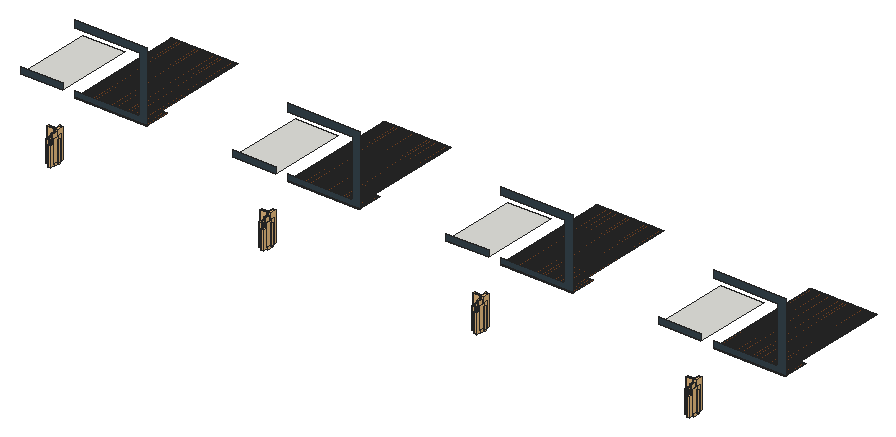
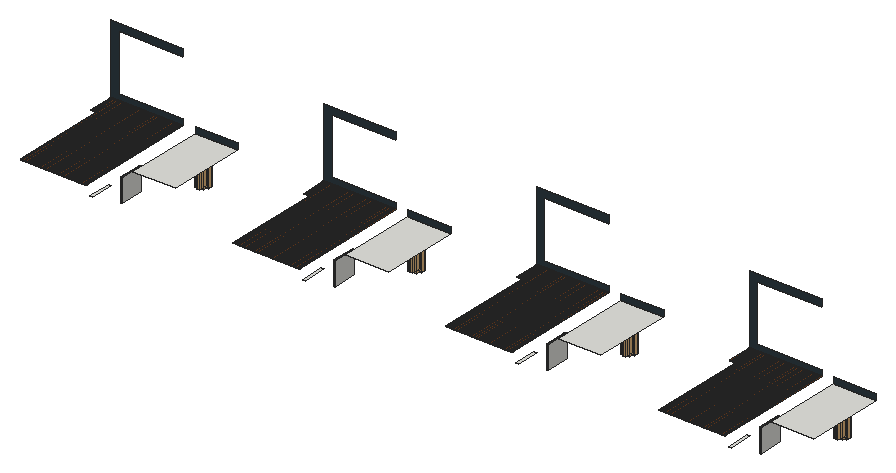
# SketchUp Ruby script. Lengths in inches.
U = 1.inch
M = Sketchup.active_model
def pt(a) = Geom::Point3d.new(a.map { |v| v * U })
def face(e, loops, mat)
  f = e.add_face(loops[0].map { |a| pt(a) })
  loops[1..].each { |l| e.add_face(l.map { |a| pt(a) }).erase! }
  f.material = f.back_material = mat if mat
  f
end
# faces: each face lists its corners as indices into pts; further lists are holes
def faces(e, pts, list, mat = nil) = list.each { |f| face(e, (f[0].is_a?(Array) ? f : [f]).map { |l| l.map { |i| pts[i] } }, mat) }
# xy, xz, yz: faces in a plane at the given z, y or x. An outline is a flat list of corners, or four numbers for a rectangle; further outlines are holes
def ring(l) = l.size == 4 ? [[l[0], l[1]], [l[2], l[1]], [l[2], l[3]], [l[0], l[3]]] : l.each_slice(2).to_a
def flat(e, list, mat, &to3) = list.each { |f| face(e, (f[0].is_a?(Array) ? f : [f]).map { |l| ring(l).map { |u, v| to3.(u, v) } }, mat) }
def xy(e, z, list, mat = nil) = flat(e, list, mat) { |x, y| [x, y, z] }
def xz(e, y, list, mat = nil) = flat(e, list, mat) { |x, z| [x, y, z] }
def yz(e, x, list, mat = nil) = flat(e, list, mat) { |y, z| [x, y, z] }
def lines(e, pts, list) = list.each { |a, b| e.add_line(pt(pts[a]), pt(pts[b])) }
# prism: a flat outline (further loops are holes) pulled along v
def prism(e, loops, v, mat = nil)
  f = face(e, loops, mat); d = Geom::Vector3d.new(v.map { |x| x * U })
  f.pushpull(f.normal.samedirection?(d) ? d.length : -d.length)
end
def box(e, o, s, mat = nil) = prism(e, [[o, [o[0] + s[0], o[1], o[2]], [o[0] + s[0], o[1] + s[1], o[2]], [o[0], o[1] + s[1], o[2]]]], [0, 0, s[2]], mat)
def at(x, y, z, deg = 0) = Geom::Transformation.translation(pt([x, y, z])) * Geom::Transformation.rotation(ORIGIN, Z_AXIS, deg.degrees)
def axes(o, x, y, z) = Geom::Transformation.new([*x, 0, *y, 0, *z, 0, *pt(o).to_a, 1])
def part(name) = M.definitions.add(name)
# library, detail: a bought-in or finely detailed component or shape, given as its bounding box
def library(name, o, s) = part(name).tap { |d| box(d.entities, o, s) }
def detail(e, o, s) = box(e.add_group.entities, o, s)
def put(e, d, t, mat = nil) = e.add_instance(d, t).tap { |i| i.material = mat if mat }
def group(e, t, mat = nil) = e.add_group.tap { |g| g.transformation = t; g.material = mat if mat }.entities
root = M.entities
M.materials.add("1480 AP K099 Starless Night-N").color = [54, 68, 77]
M.materials.add("Glass_Tinted_Gray").color = [0, 0, 0]
M.materials["Glass_Tinted_Gray"].alpha = 0.125
M.materials.add("POT_TEXTURE_1").color = [172, 172, 172]
M.materials.add("[0135_DarkGray]1").color = [81, 81, 81]
M.materials.add("[Mirror 02]").color = [229, 229, 229]
M.materials.add("[Terrazzo Light Blue]").color = [196, 214, 227]
M.materials.add("[Wood Cherry Original]").color = [152, 86, 42]
M.materials.add("white_concrete_pot1").color = [212, 211, 204]
c1 = library("Group\#12",[-312.76,2118.02,370.79],[80.37,61.43,57.53])
c2 = library("Group\#37",[-146.29,2044.53,349.125],[81,53.32,37.9])
c3 = library("Group\#85",[-236.03,2064.57,238.29],[378.97,266.89,1422.96])
c4 = library("Group\#21",[-392.38,2142.99,345.23],[79.77,60.6,39.05])
c5 = library("Group\#52",[-390.04,2074.71,363.78],[77.3,84.83,61.55])
c6 = library("Group\#25",[-389.63,2051.04,359.41],[56.81,81.38,37.86])
c7 = library("Group\#29",[-362.86,1963.26,351.01],[55.56,80.44,37.9])
c8 = library("Group\#36",[-200.52,1998.86,370.22],[77.15,68.38,35.39])
c9 = library("Group\#48",[-480.58,1843.32,11.96],[467.85,466.24,378.92])
c10 = library("Group\#22",[-433.57,2042.61,369.7],[71.79,72.8,37.85])
c11 = library("Group\#19",[-148.5,2084.1,354.63],[73.89,71.73,39.48])
c12 = library("Group\#63",[-372.4375,2154.5,374],[76.125,67.08,39.0625])
c13 = library("Group\#64",[-275.5,2156.34,352.11],[71.39,73.27,44.69])
c14 = library("Group\#42",[-143.56,2061.14,371.42],[79.79,63.19,51.3])
c15 = library("Group\#51",[-363.89,1895.22,354.63],[76.92,66.54,39.48])
c16 = library("Group\#44",[-145.08,2015.32,369.99],[82.29,54.05,37.9])
c17 = library("Group\#60",[-315.77,2202.04,371],[80.74,54.44,37.85])
c18 = library("Group\#53",[-419.21,1941.11,355.02],[73.1,71.21,39.06])
c19 = library("Group\#56",[-229.79,1894.04,351.01],[79.82,63.55,37.9])
c20 = library("Group\#70",[-234.26,2180.97,367.05],[50.63,74.65,43.95])
c21 = library("Group\#72",[-904.81,1865.01,156.3],[624.43,217.34,1227.7])
c22 = library("Group\#73",[-312.51,1611.52,263.78],[120.52,408.52,1275.1])
c23 = library("Group\#75",[-571.16,1736.08,232.33],[294.08,306.57,1438.75])
c24 = library("Group\#77",[-273.21,1593.22,47.51],[374.54,419.07,1416.6])
c25 = library("Group\#16",[-202.35,1900.5,372.29],[58.53,80.11,50.06])
c26 = library("Group\#24",[-432.01,1984.38,372.6875],[64.1,75.95,39.0625])
c27 = library("Group\#41",[-310.7,1952.62,354.63],[79.53,58.52,39.48])
c28 = library("Group\#23",[-374.28,1979.7,369.99],[51.81,82.66,37.9])
c29 = library("Group\#58",[-397.18,1916.74,372.44],[70.02,74.57,49.25])
c30 = library("Group\#66",[-236.3,2186.8,344.47],[79.26,62.91,39.06])
c31 = library("Group\#15",[-161.07,2117.49,373.61],[81.25,53.73,39.48])
c32 = library("Group\#71",[-431.9,1883.46,368.72],[373.65,376.39,18.61])
c33 = library("Group\#40",[-340.96,1970.4,361.28],[81.22,51.59,61.62])
c34 = library("Group\#46",[-272.7,1884.51,369.99],[80.39,55.87,37.9])
c35 = library("Group\#35",[-330.83,2117.69,370.2],[61.83,80.2,35.55])
c36 = library("Group\#69",[-366.3125,2177.8,359.41],[79.9,61.23,37.86])
c37 = library("Group\#28",[-435.875,2067.96,347.82],[58.32,80.53,38.29])
c38 = library("Group\#65",[-183.79,2161.45,371.25],[72.43,70.21,54.35])
c39 = library("Group\#76",[-208.23,2037.18,75.37],[621.09,225.61,1251.82])
c40 = library("Group\#79",[-675.58,1862.05,152.55],[378.81,196.01,1743.84])
c41 = library("Group\#80",[-257.06,2048.08,160.05],[394.6,177.93,1743.83])
c42 = library("Group\#82",[-344.84,1500.61,160.55],[176.35,551.19,1921.45])
c43 = library("Group\#83",[-231.77,1913.24,119.96],[448.93,143.84,1582.05])
c44 = library("Group\#84",[-616.67,2098.6,178.29],[331.19,111.16,1177.92])
c45 = library("Group\#78",[-527.15,2088.47,150.96],[267.01,328.12,1599.25])
c46 = library("Group\#87",[-792.12,2067.32,152.13],[549.56,259.52,1931.8])
c47 = library("Group\#88",[-281.17,2118.67,243.77],[133.23,408.71,1313.3])
c48 = part("Potted foliage plant")
g1 = group(c48.entities,at(904.81,-1500.61,-11.96),"white_concrete_pot1")
detail(g1,[-222.14,2117.95,372.07],[61.87,75.41,50.35])
put(c48.entities,c1,at(904.81,-1500.61,-11.96),"white_concrete_pot1")
g2 = group(c48.entities,at(904.81,-1500.61,-11.96),"white_concrete_pot1")
detail(g2,[-313.93,1881.02,351.21],[70.15,73.18,37.2])
g3 = group(c48.entities,at(904.81,-1500.61,-11.96),"white_concrete_pot1")
detail(g3,[-209.1,1970.26,378.89],[50.57,81.04,37.2])
put(c48.entities,c2,at(904.81,-1500.61,-11.96),"white_concrete_pot1")
put(c48.entities,c3,at(904.81,-1500.61,-11.96))
put(c48.entities,c4,at(904.81,-1500.61,-11.96),"white_concrete_pot1")
put(c48.entities,c5,at(904.81,-1500.61,-11.96),"white_concrete_pot1")
put(c48.entities,c6,at(904.81,-1500.61,-11.96),"white_concrete_pot1")
put(c48.entities,c7,at(904.81,-1500.61,-11.96),"white_concrete_pot1")
g4 = group(c48.entities,at(904.81,-1500.61,-11.96),"white_concrete_pot1")
detail(g4,[-129.49,1972.75,359.91],[55.59,80.76,37.2])
put(c48.entities,c8,at(904.81,-1500.61,-11.96),"white_concrete_pot1")
g5 = group(c48.entities,at(904.81,-1500.61,-11.96),"white_concrete_pot1")
detail(g5,[-333.13,1892.25,370.19],[61.39,79.4,37.2])
put(c48.entities,c9,at(904.81,-1500.61,-11.96),"POT_TEXTURE_1")
put(c48.entities,c10,at(904.81,-1500.61,-11.96),"white_concrete_pot1")
put(c48.entities,c11,at(904.81,-1500.61,-11.96),"white_concrete_pot1")
g6 = group(c48.entities,at(904.81,-1500.61,-11.96),"white_concrete_pot1")
detail(g6,[-270.91,2176.57,345.18],[52.11,82.01,38.29])
g7 = group(c48.entities,at(904.81,-1500.61,-11.96),"white_concrete_pot1")
detail(g7,[-195.71,2019.1875,371.11],[58.98,81.18,37.2])
g8 = group(c48.entities,at(904.81,-1500.61,-11.96),"white_concrete_pot1")
detail(g8,[-319.36,2078.81,339.18],[76.07,69.08,39.48])
put(c48.entities,c12,at(904.81,-1500.61,-11.96),"white_concrete_pot1")
put(c48.entities,c13,at(904.81,-1500.61,-11.96),"white_concrete_pot1")
g9 = group(c48.entities,at(904.81,-1500.61,-11.96),"white_concrete_pot1")
detail(g9,[-417.64,2112.53,369.82],[65.44,79.59,38.29])
put(c48.entities,c14,at(904.81,-1500.61,-11.96),"white_concrete_pot1")
put(c48.entities,c15,at(904.81,-1500.61,-11.96),"white_concrete_pot1")
put(c48.entities,c16,at(904.81,-1500.61,-11.96),"white_concrete_pot1")
g10 = group(c48.entities,at(904.81,-1500.61,-11.96),"white_concrete_pot1")
detail(g10,[-240.6,2054.85,378.89],[71.5,72.03,37.2])
put(c48.entities,c17,at(904.81,-1500.61,-11.96),"white_concrete_pot1")
put(c48.entities,c18,at(904.81,-1500.61,-11.96),"white_concrete_pot1")
put(c48.entities,c19,at(904.81,-1500.61,-11.96),"white_concrete_pot1")
g11 = group(c48.entities,at(904.81,-1500.61,-11.96),"white_concrete_pot1")
detail(g11,[-249.82,2117.53,359.91],[58.07,81.25,37.2])
put(c48.entities,c20,at(904.81,-1500.61,-11.96),"white_concrete_pot1")
put(c48.entities,c21,at(904.81,-1500.61,-11.96))
put(c48.entities,c22,at(904.81,-1500.61,-11.96))
put(c48.entities,c23,at(904.81,-1500.61,-11.96))
put(c48.entities,c24,at(904.81,-1500.61,-11.96))
g12 = group(c48.entities,at(904.81,-1500.61,-11.96),"white_concrete_pot1")
detail(g12,[-435.4375,2027.54,350.71],[78.74,62.6,37.86])
put(c48.entities,c25,at(904.81,-1500.61,-11.96),"white_concrete_pot1")
g13 = group(c48.entities,at(904.81,-1500.61,-11.96),"white_concrete_pot1")
detail(g13,[-173.8,2126.25,354.63],[80.17,60.53,39.48])
g14 = group(c48.entities,at(904.81,-1500.61,-11.96),"white_concrete_pot1")
detail(g14,[-222.96,2066.75,359.91],[63.77,78.21,37.2])
put(c48.entities,c26,at(904.81,-1500.61,-11.96),"white_concrete_pot1")
g15 = group(c48.entities,at(904.81,-1500.61,-11.96),"white_concrete_pot1")
detail(g15,[-183.125,1913.38,330.04],[66.78,77.69,39.48])
put(c48.entities,c27,at(904.81,-1500.61,-11.96),"white_concrete_pot1")
g16 = group(c48.entities,at(904.81,-1500.61,-11.96),"white_concrete_pot1")
detail(g16,[-152,1936.85,378.89],[64.46,79.76,37.2])
g17 = group(c48.entities,at(904.81,-1500.61,-11.96),"white_concrete_pot1")
detail(g17,[-284.65,1933.22,373.64],[80.83,55.23,37.2])
put(c48.entities,c28,at(904.81,-1500.61,-11.96),"white_concrete_pot1")
g18 = group(c48.entities,at(904.81,-1500.61,-11.96),"white_concrete_pot1")
detail(g18,[-263.49,1923.54,359.91],[75.98,66.75,37.2])
put(c48.entities,c29,at(904.81,-1500.61,-11.96),"white_concrete_pot1")
g19 = group(c48.entities,at(904.81,-1500.61,-11.96),"white_concrete_pot1")
detail(g19,[-167.97,1940.97,354.63],[66.78,77.7,39.48])
put(c48.entities,c30,at(904.81,-1500.61,-11.96),"white_concrete_pot1")
g20 = group(c48.entities,at(904.81,-1500.61,-11.96),"white_concrete_pot1")
detail(g20,[-214.75,1956.59,330.04],[66.78,77.69,39.48])
put(c48.entities,c31,at(904.81,-1500.61,-11.96),"white_concrete_pot1")
put(c48.entities,c32,at(904.81,-1500.61,-11.96),"white_concrete_pot1")
put(c48.entities,c33,at(904.81,-1500.61,-11.96),"white_concrete_pot1")
g21 = group(c48.entities,at(904.81,-1500.61,-11.96),"white_concrete_pot1")
detail(g21,[-282.5625,1934.21,389.56],[81.1,59.19,35.03])
put(c48.entities,c34,at(904.81,-1500.61,-11.96),"white_concrete_pot1")
g22 = group(c48.entities,at(904.81,-1500.61,-11.96),"white_concrete_pot1")
detail(g22,[-394.5,2036.48,359.91],[79.58,64.84,37.2])
put(c48.entities,c35,at(904.81,-1500.61,-11.96),"white_concrete_pot1")
put(c48.entities,c36,at(904.81,-1500.61,-11.96),"white_concrete_pot1")
put(c48.entities,c37,at(904.81,-1500.61,-11.96),"white_concrete_pot1")
put(c48.entities,c38,at(904.81,-1500.61,-11.96),"white_concrete_pot1")
put(c48.entities,c39,at(904.81,-1500.61,-11.96))
put(c48.entities,c40,at(904.81,-1500.61,-11.96))
put(c48.entities,c41,at(904.81,-1500.61,-11.96))
put(c48.entities,c42,at(904.81,-1500.61,-11.96))
put(c48.entities,c43,at(904.81,-1500.61,-11.96))
put(c48.entities,c44,at(904.81,-1500.61,-11.96))
put(c48.entities,c45,at(904.81,-1500.61,-11.96))
put(c48.entities,c46,at(904.81,-1500.61,-11.96))
put(c48.entities,c47,at(904.81,-1500.61,-11.96))
c49 = part("PENTEK_RP Fineline 50S_Sliding_DoorCase_E1")
box(c49.entities,[0,0,0],[1.51,3.66,99.27],"[0135_DarkGray]1")
c50 = part("PENTEK_RP Fineline 50S_SlidingDooe_Case_E2")
box(c50.entities,[0,0,0],[96.25,3.66,1.51],"[0135_DarkGray]1")
c51 = part("pentek_RP Fineline 50S_SlidingDoor_Case")
put(c51.entities,c49,at(97.76,0,0))
put(c51.entities,c50,at(1.51,0,0))
put(c51.entities,c49,at(0,0,0))
put(c51.entities,c50,at(1.51,0,97.76))
c52 = part("PENTEK_RP Fineline 50S_SlidingDoor_GlazingBead_2")
box(c52.entities,[0,0,0],[0.56,0.59,94.39],"[0135_DarkGray]1")
c53 = part("PENTEK_RP Fineline 50S_SlidingDoor_Glass")
box(c53.entities,[0,0,0],[46.58,0.16,94.39],"Glass_Tinted_Gray")
c54 = part("PENTEK_RP Fineline 50S_SlidingDoor_GlazingBead")
box(c54.entities,[0,0,0],[45.47,0.59,0.56],"[0135_DarkGray]1")
c55 = part("PENTEK_RP Fineline 50S_SlidingDoor_Leaf_E1")
xy(c55.entities,0,[[0,0,0.93,1.97],[0.93,1.57,1.49,1.97]],"[0135_DarkGray]1")
xy(c55.entities,96.25,[[0,0,0.93,0,0.93,1.57,1.49,1.57,1.49,1.97,0,1.97]],"[0135_DarkGray]1")
xz(c55.entities,0,[[0,0,0.93,96.25]],"[0135_DarkGray]1")
xz(c55.entities,1.57,[[0.93,0,1.49,95.32],[0.93,95.32,1.49,96.25]],"[0135_DarkGray]1")
xz(c55.entities,1.97,[[0,0,1.49,96.25]],"[0135_DarkGray]1")
yz(c55.entities,0,[[0,0,1.97,96.25]],"[0135_DarkGray]1")
yz(c55.entities,0.93,[[0,0,1.57,0.93],[0,0.93,1.57,95.32],[0,95.32,1.57,96.25]],"[0135_DarkGray]1")
yz(c55.entities,1.49,[[1.57,0,1.97,95.32],[1.57,95.32,1.97,96.25]],"[0135_DarkGray]1")
c56 = part("PENTEK_RP Fineline 50S_SlidingDoor_Leaf_E2")
xy(c56.entities,0,[[0,0,0,1.57,0.56,1.57,0.56,1.97,46.02,1.97,46.02,1.57,46.58,1.57,46.58,0]],"[0135_DarkGray]1")
xy(c56.entities,0.93,[[0,0,46.58,1.57]],"[0135_DarkGray]1")
xy(c56.entities,1.49,[[0.56,1.57,46.02,1.97]],"[0135_DarkGray]1")
xz(c56.entities,0,[[0,0,46.58,0.93]],"[0135_DarkGray]1")
xz(c56.entities,1.57,[[0,0,0.56,0.93],[46.02,0,46.58,0.93],[0.56,0.93,46.02,1.49]],"[0135_DarkGray]1")
xz(c56.entities,1.97,[[0.56,0,46.02,1.49]],"[0135_DarkGray]1")
yz(c56.entities,0,[[0,0,1.57,0.93]],"[0135_DarkGray]1")
yz(c56.entities,0.56,[[1.57,0,1.97,0.93],[1.57,0.93,1.97,1.49]],"[0135_DarkGray]1")
yz(c56.entities,46.02,[[1.57,0,1.97,0.93],[1.57,0.93,1.97,1.49]],"[0135_DarkGray]1")
yz(c56.entities,46.58,[[0,0,1.57,0.93]],"[0135_DarkGray]1")
c57 = part("PENTEK_RP Fineline S_SlidingDoor_Leaf1")
put(c57.entities,c52,at(0.93,0,0.93))
put(c57.entities,c52,at(46.96,0,0.93))
put(c57.entities,c53,at(1.49,1.42,0.93))
put(c57.entities,c54,at(1.49,0,0.93))
put(c57.entities,c53,at(1.49,0.59,0.93),"[Terrazzo Light Blue]")
put(c57.entities,c55,at(0,0,0))
put(c57.entities,c55,axes([48.44,0,0],[-1,0,0],[0,1,0],[0,0,1]))
put(c57.entities,c56,axes([0.93,0,96.25],[1,0,0],[0,1,0],[0,0,-1]))
put(c57.entities,c56,at(0.93,0,0))
put(c57.entities,c54,at(1.49,0,94.77))
c58 = part("PENTEK_RP Fineline 50S_SlidingDoor_Leaf2")
put(c58.entities,c53,at(1.49,1.42,0.93))
put(c58.entities,c54,at(1.49,0,94.77))
put(c58.entities,c52,at(46.96,0,0.93))
put(c58.entities,c53,at(1.49,0.59,0.93),"[Mirror 02]")
put(c58.entities,c52,at(0.93,0,0.93))
put(c58.entities,c55,at(0,0,0))
put(c58.entities,c55,axes([48.44,0,0],[-1,0,0],[0,1,0],[0,0,1]))
put(c58.entities,c54,at(1.49,0,0.93))
put(c58.entities,c56,axes([0.93,0,96.25],[1,0,0],[0,1,0],[0,0,-1]))
put(c58.entities,c56,at(0.93,0,0))
c59 = part("PENTEK - Slimmest Steel Sliding Door / Window\#1")
put(c59.entities,c51,at(0,-1.88,-0.09))
put(c59.entities,c57,at(1.51,-2.27,1.42))
put(c59.entities,c58,at(49.32,-0.3,1.42))
c60 = part("Group50\#1")
box(c60.entities,[-75,-126,0],[1.18,252,0.24])
c61 = part("Group51\#1")
box(c61.entities,[-73.62,-126,0],[1.18,252,0.24])
c62 = part("Group52\#1")
box(c62.entities,[-72.24,-126,0],[1.18,252,0.24])
c63 = part("Group53\#1")
box(c63.entities,[-70.87,-126,0],[1.18,252,0.24])
c64 = part("Group54\#1")
box(c64.entities,[-69.49,-126,0],[1.18,252,0.24])
c65 = part("Group55\#1")
box(c65.entities,[-68.11,-126,0],[1.18,252,0.24])
c66 = part("Group56\#1")
box(c66.entities,[-66.73,-126,0],[1.18,252,0.24])
c67 = part("Group57\#1")
box(c67.entities,[-65.35,-126,0],[1.18,252,0.24])
c68 = part("Group58\#1")
box(c68.entities,[-63.98,-126,0],[1.18,252,0.24])
c69 = part("Group59\#1")
box(c69.entities,[-62.6,-126,0],[1.18,252,0.24])
c70 = part("Group60\#1")
box(c70.entities,[-61.22,-126,0],[1.18,252,0.24])
c71 = part("Group61\#1")
box(c71.entities,[-59.84,-126,0],[1.18,252,0.24])
c72 = part("Group62\#1")
box(c72.entities,[-58.46,-126,0],[1.18,252,0.24])
c73 = part("Group63\#1")
box(c73.entities,[-57.09,-126,0],[1.18,252,0.24])
c74 = part("Group64\#1")
box(c74.entities,[-55.71,-126,0],[1.18,252,0.24])
c75 = part("Group65\#1")
box(c75.entities,[-54.33,-126,0],[1.18,252,0.24])
c76 = part("Group66\#1")
box(c76.entities,[-52.95,-126,0],[1.18,252,0.24])
c77 = part("Group67\#1")
box(c77.entities,[-51.57,-126,0],[1.18,252,0.24])
c78 = part("Group68\#1")
box(c78.entities,[-50.2,-126,0],[1.18,252,0.24])
c79 = part("Group69\#1")
box(c79.entities,[-48.82,-126,0],[1.18,252,0.24])
c80 = part("Group70\#1")
box(c80.entities,[-47.44,-126,0],[1.18,252,0.24])
c81 = part("Group71\#1")
box(c81.entities,[-46.0625,-126,0],[1.18,252,0.24])
c82 = part("Group72\#1")
box(c82.entities,[-44.69,-126,0],[1.19,252,0.24])
c83 = part("Group73\#1")
box(c83.entities,[-43.31,-126,0],[1.19,252,0.24])
c84 = part("Group74\#1")
box(c84.entities,[-41.93,-126,0],[1.18,252,0.24])
c85 = part("Group75\#1")
box(c85.entities,[-40.55,-126,0],[1.18,252,0.24])
c86 = part("Group76\#1")
box(c86.entities,[-39.17,-126,0],[1.18,252,0.24])
c87 = part("Group77\#1")
box(c87.entities,[-37.8,-126,0],[1.19,252,0.24])
c88 = part("Group78\#1")
box(c88.entities,[-36.42,-126,0],[1.18,252,0.24])
c89 = part("Group79\#1")
box(c89.entities,[-35.04,-126,0],[1.18,252,0.24])
c90 = part("Group80\#1")
box(c90.entities,[-33.66,-126,0],[1.18,252,0.24])
c91 = part("Group81\#1")
box(c91.entities,[-32.28,-126,0],[1.18,252,0.24])
c92 = part("Group82\#1")
box(c92.entities,[-30.91,-126,0],[1.19,252,0.24])
c93 = part("Group83\#1")
box(c93.entities,[-29.53,-126,0],[1.18,252,0.24])
c94 = part("Group84\#1")
box(c94.entities,[-28.15,-126,0],[1.18,252,0.24])
c95 = part("Group85\#1")
box(c95.entities,[-26.77,-126,0],[1.18,252,0.24])
c96 = part("Group86\#1")
box(c96.entities,[-25.39,-126,0],[1.18,252,0.24])
c97 = part("Group87\#1")
box(c97.entities,[-24.02,-126,0],[1.19,252,0.24])
c98 = part("Group88\#1")
box(c98.entities,[-22.64,-126,0],[1.18,252,0.24])
c99 = part("Group89\#1")
box(c99.entities,[-21.26,-126,0],[1.18,252,0.24])
c100 = part("Group90\#1")
box(c100.entities,[-19.88,-126,0],[1.18,252,0.24])
c101 = part("Group91\#1")
box(c101.entities,[-18.5,-126,0],[1.18,252,0.24])
c102 = part("Group92\#1")
box(c102.entities,[-17.125,-126,0],[1.19,252,0.24])
c103 = part("Group93\#1")
box(c103.entities,[-15.75,-126,0],[1.18,252,0.24])
c104 = part("Group94\#1")
box(c104.entities,[-14.37,-126,0],[1.18,252,0.24])
c105 = part("Group95\#1")
box(c105.entities,[-12.99,-126,0],[1.18,252,0.24])
c106 = part("Group96\#1")
box(c106.entities,[-11.61,-126,0],[1.18,252,0.24])
c107 = part("Group97\#1")
box(c107.entities,[-10.24,-126,0],[1.18,252,0.24])
c108 = part("Group98\#1")
box(c108.entities,[-8.86,-126,0],[1.18,252,0.24])
c109 = part("Group99\#1")
box(c109.entities,[-7.48,-126,0],[1.18,252,0.24])
c110 = part("Group100\#1")
box(c110.entities,[-6.1,-126,0],[1.18,252,0.24])
c111 = part("Group101\#1")
box(c111.entities,[-4.72,-126,0],[1.18,252,0.24])
c112 = part("Group102\#1")
box(c112.entities,[-3.35,-126,0],[1.18,252,0.24])
c113 = part("Group103\#1")
box(c113.entities,[-1.97,-126,0],[1.18,252,0.24])
c114 = part("Group104\#1")
box(c114.entities,[-0.59,-126,0],[1.18,252,0.24])
c115 = part("Group105\#1")
box(c115.entities,[0.79,-126,0],[1.18,252,0.24])
c116 = part("Group106\#1")
box(c116.entities,[2.17,-126,0],[1.18,252,0.24])
c117 = part("Group107\#1")
box(c117.entities,[3.54,-126,0],[1.18,252,0.24])
c118 = part("Group108\#1")
box(c118.entities,[4.92,-126,0],[1.18,252,0.24])
c119 = part("Group109\#1")
box(c119.entities,[6.3,-126,0],[1.18,252,0.24])
c120 = part("Group110\#1")
box(c120.entities,[7.68,-126,0],[1.18,252,0.24])
c121 = part("Group111\#1")
box(c121.entities,[9.06,-126,0],[1.18,252,0.24])
c122 = part("Group112\#1")
box(c122.entities,[10.43,-126,0],[1.18,252,0.24])
c123 = part("Group113\#1")
box(c123.entities,[11.8125,-126,0],[1.18,252,0.24])
c124 = part("Group114\#1")
box(c124.entities,[13.1875,-126,0],[1.18,252,0.24])
c125 = part("Group115\#1")
box(c125.entities,[14.57,-126,0],[1.18,252,0.24])
c126 = part("Group116\#1")
box(c126.entities,[15.94,-126,0],[1.19,252,0.24])
c127 = part("Group117\#1")
box(c127.entities,[17.32,-126,0],[1.18,252,0.24])
c128 = part("Group118\#1")
box(c128.entities,[18.7,-126,0],[1.18,252,0.24])
c129 = part("Group119\#1")
box(c129.entities,[20.08,-126,0],[1.18,252,0.24])
c130 = part("Group120\#1")
box(c130.entities,[21.46,-126,0],[1.18,252,0.24])
c131 = part("Group121\#1")
box(c131.entities,[22.83,-126,0],[1.19,252,0.24])
c132 = part("Group122\#1")
box(c132.entities,[24.21,-126,0],[1.18,252,0.24])
c133 = part("Group123\#1")
box(c133.entities,[25.59,-126,0],[1.18,252,0.24])
c134 = part("Group124\#1")
box(c134.entities,[26.97,-126,0],[1.18,252,0.24])
c135 = part("Group125\#1")
box(c135.entities,[28.35,-126,0],[1.18,252,0.24])
c136 = part("Group126\#1")
box(c136.entities,[29.72,-126,0],[1.19,252,0.24])
c137 = part("Group127\#1")
box(c137.entities,[31.1,-126,0],[1.18,252,0.24])
c138 = part("Group128\#1")
box(c138.entities,[32.48,-126,0],[1.18,252,0.24])
c139 = part("Group129\#1")
box(c139.entities,[33.86,-126,0],[1.18,252,0.24])
c140 = part("Group130\#1")
box(c140.entities,[35.24,-126,0],[1.18,252,0.24])
c141 = part("Group131\#1")
box(c141.entities,[36.61,-126,0],[1.19,252,0.24])
c142 = part("Group132\#1")
box(c142.entities,[37.99,-126,0],[1.18,252,0.24])
c143 = part("Group133\#1")
box(c143.entities,[39.37,-126,0],[1.18,252,0.24])
c144 = part("Group134\#1")
box(c144.entities,[40.75,-126,0],[1.18,252,0.24])
c145 = part("Group135\#1")
box(c145.entities,[42.125,-126,0],[1.19,252,0.24])
c146 = part("Group136\#1")
box(c146.entities,[43.5,-126,0],[1.19,252,0.24])
c147 = part("Group137\#1")
box(c147.entities,[44.88,-126,0],[1.18,252,0.24])
c148 = part("Group138\#1")
box(c148.entities,[46.26,-126,0],[1.18,252,0.24])
c149 = part("Group139\#1")
box(c149.entities,[47.64,-126,0],[1.18,252,0.24])
c150 = part("Group140\#1")
box(c150.entities,[49.02,-126,0],[1.18,252,0.24])
c151 = part("Group141\#2")
box(c151.entities,[50.39,-126,0],[1.18,252,0.24])
c152 = part("Group142\#1")
box(c152.entities,[51.77,-126,0],[1.18,252,0.24])
c153 = part("Group143\#1")
box(c153.entities,[53.15,-126,0],[1.18,252,0.24])
c154 = part("Group144\#2")
box(c154.entities,[54.53,-126,0],[1.18,252,0.24])
c155 = part("Group145\#1")
box(c155.entities,[55.91,-126,0],[1.18,252,0.24])
c156 = part("Group146\#1")
box(c156.entities,[57.28,-126,0],[1.18,252,0.24])
c157 = part("Group147\#1")
box(c157.entities,[58.66,-126,0],[1.18,252,0.24])
c158 = part("Group148\#1")
box(c158.entities,[60.04,-126,0],[1.18,252,0.24])
c159 = part("Group149\#1")
box(c159.entities,[61.42,-126,0],[1.18,252,0.24])
c160 = part("Group150\#1")
xy(c160.entities,0,[[62.8,-126,62.8,126,63,126,63,-73.9375,63.98,-73.9375,63.98,-126]])
xy(c160.entities,0.24,[[62.8,-126,63.98,-126,63.98,-73.9375,63,-73.9375,63,126,62.8,126]])
xz(c160.entities,-126,[[62.8,0,63.98,0.24]])
yz(c160.entities,62.8,[[-126,0,126,0.24]])
yz(c160.entities,63.98,[[-126,0,-73.9375,0.24]])
c161 = part("Group151\#1")
box(c161.entities,[64.17,-126,0],[1.18,52.0625,0.24])
c162 = part("Group152\#1")
box(c162.entities,[65.55,-126,0],[1.18,52.0625,0.24])
c163 = part("Group153\#1")
box(c163.entities,[66.93,-126,0],[1.18,52.0625,0.24])
c164 = part("Group154\#1")
box(c164.entities,[68.31,-126,0],[1.18,52.0625,0.24])
c165 = part("Group155\#1")
box(c165.entities,[69.69,-126,0],[1.18,52.0625,0.24])
c166 = part("Group156\#1")
box(c166.entities,[71.0625,-126,0],[1.18,52.0625,0.24])
c167 = part("Group157\#1")
box(c167.entities,[72.44,-126,0],[1.18,52.0625,0.24])
c168 = part("Group158\#1")
box(c168.entities,[73.82,-126,0],[1.18,52.0625,0.24])
c169 = part("Group48\#1")
put(c169.entities,c60,at(0,0,0))
put(c169.entities,c61,at(0,0,0))
put(c169.entities,c62,at(0,0,0))
put(c169.entities,c63,at(0,0,0))
put(c169.entities,c64,at(0,0,0))
put(c169.entities,c65,at(0,0,0))
put(c169.entities,c66,at(0,0,0))
put(c169.entities,c67,at(0,0,0))
put(c169.entities,c68,at(0,0,0))
put(c169.entities,c69,at(0,0,0))
put(c169.entities,c70,at(0,0,0))
put(c169.entities,c71,at(0,0,0))
put(c169.entities,c72,at(0,0,0))
put(c169.entities,c73,at(0,0,0))
put(c169.entities,c74,at(0,0,0))
put(c169.entities,c75,at(0,0,0))
put(c169.entities,c76,at(0,0,0))
put(c169.entities,c77,at(0,0,0))
put(c169.entities,c78,at(0,0,0))
put(c169.entities,c79,at(0,0,0))
put(c169.entities,c80,at(0,0,0))
put(c169.entities,c81,at(0,0,0))
put(c169.entities,c82,at(0,0,0))
put(c169.entities,c83,at(0,0,0))
put(c169.entities,c84,at(0,0,0))
put(c169.entities,c85,at(0,0,0))
put(c169.entities,c86,at(0,0,0))
put(c169.entities,c87,at(0,0,0))
put(c169.entities,c88,at(0,0,0))
put(c169.entities,c89,at(0,0,0))
put(c169.entities,c90,at(0,0,0))
put(c169.entities,c91,at(0,0,0))
put(c169.entities,c92,at(0,0,0))
put(c169.entities,c93,at(0,0,0))
put(c169.entities,c94,at(0,0,0))
put(c169.entities,c95,at(0,0,0))
put(c169.entities,c96,at(0,0,0))
put(c169.entities,c97,at(0,0,0))
put(c169.entities,c98,at(0,0,0))
put(c169.entities,c99,at(0,0,0))
put(c169.entities,c100,at(0,0,0))
put(c169.entities,c101,at(0,0,0))
put(c169.entities,c102,at(0,0,0))
put(c169.entities,c103,at(0,0,0))
put(c169.entities,c104,at(0,0,0))
put(c169.entities,c105,at(0,0,0))
put(c169.entities,c106,at(0,0,0))
put(c169.entities,c107,at(0,0,0))
put(c169.entities,c108,at(0,0,0))
put(c169.entities,c109,at(0,0,0))
put(c169.entities,c110,at(0,0,0))
put(c169.entities,c111,at(0,0,0))
put(c169.entities,c112,at(0,0,0))
put(c169.entities,c113,at(0,0,0))
put(c169.entities,c114,at(0,0,0))
put(c169.entities,c115,at(0,0,0))
put(c169.entities,c116,at(0,0,0))
put(c169.entities,c117,at(0,0,0))
put(c169.entities,c118,at(0,0,0))
put(c169.entities,c119,at(0,0,0))
put(c169.entities,c120,at(0,0,0))
put(c169.entities,c121,at(0,0,0))
put(c169.entities,c122,at(0,0,0))
put(c169.entities,c123,at(0,0,0))
put(c169.entities,c124,at(0,0,0))
put(c169.entities,c125,at(0,0,0))
put(c169.entities,c126,at(0,0,0))
put(c169.entities,c127,at(0,0,0))
put(c169.entities,c128,at(0,0,0))
put(c169.entities,c129,at(0,0,0))
put(c169.entities,c130,at(0,0,0))
put(c169.entities,c131,at(0,0,0))
put(c169.entities,c132,at(0,0,0))
put(c169.entities,c133,at(0,0,0))
put(c169.entities,c134,at(0,0,0))
put(c169.entities,c135,at(0,0,0))
put(c169.entities,c136,at(0,0,0))
put(c169.entities,c137,at(0,0,0))
put(c169.entities,c138,at(0,0,0))
put(c169.entities,c139,at(0,0,0))
put(c169.entities,c140,at(0,0,0))
put(c169.entities,c141,at(0,0,0))
put(c169.entities,c142,at(0,0,0))
put(c169.entities,c143,at(0,0,0))
put(c169.entities,c144,at(0,0,0))
put(c169.entities,c145,at(0,0,0))
put(c169.entities,c146,at(0,0,0))
put(c169.entities,c147,at(0,0,0))
put(c169.entities,c148,at(0,0,0))
put(c169.entities,c149,at(0,0,0))
put(c169.entities,c150,at(0,0,0))
put(c169.entities,c151,at(0,0,0))
put(c169.entities,c152,at(0,0,0))
put(c169.entities,c153,at(0,0,0))
put(c169.entities,c154,at(0,0,0))
put(c169.entities,c155,at(0,0,0))
put(c169.entities,c156,at(0,0,0))
put(c169.entities,c157,at(0,0,0))
put(c169.entities,c158,at(0,0,0))
put(c169.entities,c159,at(0,0,0))
put(c169.entities,c160,at(0,0,0))
put(c169.entities,c161,at(0,0,0))
put(c169.entities,c162,at(0,0,0))
put(c169.entities,c163,at(0,0,0))
put(c169.entities,c164,at(0,0,0))
put(c169.entities,c165,at(0,0,0))
put(c169.entities,c166,at(0,0,0))
put(c169.entities,c167,at(0,0,0))
put(c169.entities,c168,at(0,0,0))
xy(root,54,[[291,342.875,294,390.875],[735,342.875,738,390.875],[1179,342.875,1182,390.875],[1623,342.875,1626,390.875]])
xy(root,102,[[291,342.875,294,390.875],[735,342.875,738,390.875],[1179,342.875,1182,390.875],[1623,342.875,1626,390.875],[288,424.1875,294,472.1875],
  [732,424.1875,738,472.1875],[1176,424.1875,1182,472.1875],[1620,424.1875,1626,472.1875]])
xy(root,126,[[175,236.25,263,398.125],[619,236.25,707,398.125],[1063,236.25,1151,398.125],[1507,236.25,1595,398.125]])
xz(root,229.25,[[294,126,444,126,444,271,294,271,294,256,429,256,429,139,294,139],[738,126,888,126,888,271,738,271,738,256,873,256,873,139,738,139],[1182,126,1332,126,1332,271,1182,271,1182,256,1317,256,1317,139,1182,139],[1626,126,1776,126,1776,271,1626,271,1626,256,1761,256,1761,139,1626,139]],"1480 AP K099 Starless Night-N")
xz(root,236.25,[[175,126,263,139],[619,126,707,139],[1063,126,1151,139],[1507,126,1595,139]],"1480 AP K099 Starless Night-N")
xz(root,342.875,[[291,54,294,102],[735,54,738,102],[1179,54,1182,102],[1623,54,1626,102]])
xz(root,390.875,[[291,54,294,102],[735,54,738,102],[1179,54,1182,102],[1623,54,1626,102]])
yz(root,291,[[342.875,54,390.875,102]])
yz(root,735,[[342.875,54,390.875,102]])
yz(root,1179,[[342.875,54,390.875,102]])
yz(root,1623,[[342.875,54,390.875,102]])
put(root,c48,axes([259.6875,218.51,6.53],[0,-0.0242,0],[0.0242,0,0],[0,0,0.03194]))
put(root,c48,axes([703.6875,218.51,6.53],[0,-0.0242,0],[0.0242,0,0],[0,0,0.03194]))
put(root,c48,axes([1147.6875,218.51,6.53],[0,-0.0242,0],[0.0242,0,0],[0,0,0.03194]))
put(root,c48,axes([1591.6875,218.51,6.53],[0,-0.0242,0],[0.0242,0,0],[0,0,0.03194]))
put(root,c59,axes([292.8,342.875,54.04],[0,0.48877,0],[-0.53,0,0],[0,0,0.48352]))
put(root,c59,axes([736.8,342.875,54.04],[0,0.48877,0],[-0.53,0,0],[0,0,0.48352]))
put(root,c59,axes([1180.8,342.875,54.04],[0,0.48877,0],[-0.53,0,0],[0,0,0.48352]))
put(root,c59,axes([1624.8,342.875,54.04],[0,0.48877,0],[-0.53,0,0],[0,0,0.48352]))
put(root,c169,at(369,355.25,126),"[Wood Cherry Original]")
put(root,c169,at(813,355.25,126),"[Wood Cherry Original]")
put(root,c169,at(1257,355.25,126),"[Wood Cherry Original]")
put(root,c169,at(1701,355.25,126),"[Wood Cherry Original]")
